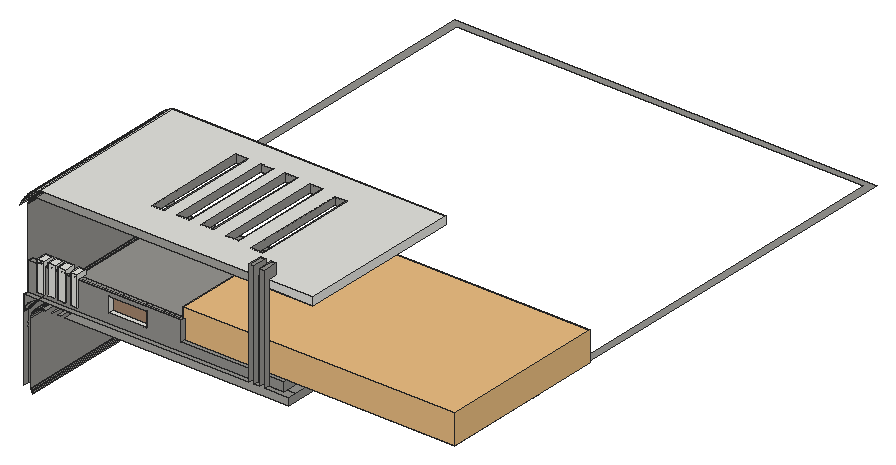
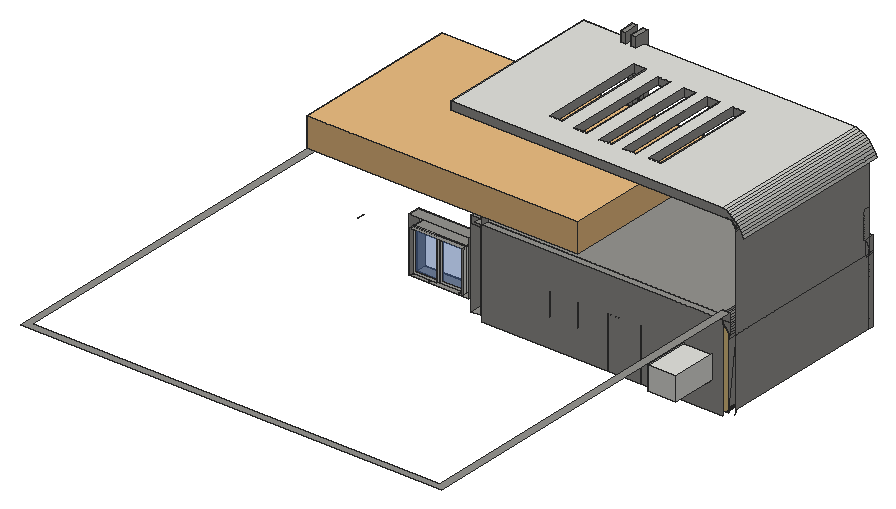
# SketchUp Ruby script. Lengths in millimetres.
U = 1.mm
M = Sketchup.active_model
def pt(a) = Geom::Point3d.new(a.map { |v| v * U })
def face(e, loops, mat)
  f = e.add_face(loops[0].map { |a| pt(a) })
  loops[1..].each { |l| e.add_face(l.map { |a| pt(a) }).erase! }
  f.material = f.back_material = mat if mat
  f
end
# faces: each face lists its corners as indices into pts; further lists are holes
def faces(e, pts, list, mat = nil) = list.each { |f| face(e, (f[0].is_a?(Array) ? f : [f]).map { |l| l.map { |i| pts[i] } }, mat) }
# xy, xz, yz: faces in a plane at the given z, y or x. An outline is a flat list of corners, or four numbers for a rectangle; further outlines are holes
def ring(l) = l.size == 4 ? [[l[0], l[1]], [l[2], l[1]], [l[2], l[3]], [l[0], l[3]]] : l.each_slice(2).to_a
def flat(e, list, mat, &to3) = list.each { |f| face(e, (f[0].is_a?(Array) ? f : [f]).map { |l| ring(l).map { |u, v| to3.(u, v) } }, mat) }
def xy(e, z, list, mat = nil) = flat(e, list, mat) { |x, y| [x, y, z] }
def xz(e, y, list, mat = nil) = flat(e, list, mat) { |x, z| [x, y, z] }
def yz(e, x, list, mat = nil) = flat(e, list, mat) { |y, z| [x, y, z] }
def lines(e, pts, list) = list.each { |a, b| e.add_line(pt(pts[a]), pt(pts[b])) }
# prism: a flat outline (further loops are holes) pulled along v
def prism(e, loops, v, mat = nil)
  f = face(e, loops, mat); d = Geom::Vector3d.new(v.map { |x| x * U })
  f.pushpull(f.normal.samedirection?(d) ? d.length : -d.length)
end
def box(e, o, s, mat = nil) = prism(e, [[o, [o[0] + s[0], o[1], o[2]], [o[0] + s[0], o[1] + s[1], o[2]], [o[0], o[1] + s[1], o[2]]]], [0, 0, s[2]], mat)
def at(x, y, z, deg = 0) = Geom::Transformation.translation(pt([x, y, z])) * Geom::Transformation.rotation(ORIGIN, Z_AXIS, deg.degrees)
def axes(o, x, y, z) = Geom::Transformation.new([*x, 0, *y, 0, *z, 0, *pt(o).to_a, 1])
def part(name) = M.definitions.add(name)
# library, detail: a bought-in or finely detailed component or shape, given as its bounding box
def library(name, o, s) = part(name).tap { |d| box(d.entities, o, s) }
def detail(e, o, s) = box(e.add_group.entities, o, s)
def put(e, d, t, mat = nil) = e.add_instance(d, t).tap { |i| i.material = mat if mat }
def group(e, t, mat = nil) = e.add_group.tap { |g| g.transformation = t; g.material = mat if mat }.entities
root = M.entities
M.materials.add("Polis06_194").color = [79, 50, 36]
M.materials.add("Teddy_BraceletShadow ").color = [165, 134, 109]
M.materials.add("[Granite Light Gray]").color = [149, 148, 144]
M.materials.add("[Stone Brushed Khaki]").color = [226, 197, 133]
M.materials.add("[Translucent Glass Blue]").color = [100, 149, 237]
M.materials["[Translucent Glass Blue]"].alpha = 0.5
c1 = part("Flush door")
xy(c1.entities,0,[[0,0,120,30],[0,870,120,900]],"Polis06_194")
xy(c1.entities,2165.6,[[0,30,120,870]],"Polis06_194")
xy(c1.entities,2200,[[0,0,120,900]],"Polis06_194")
xz(c1.entities,0,[[0,0,120,2200]],"Polis06_194")
xz(c1.entities,30,[[0,0,60,2165.6],[60,0,120,2165.6]],"Polis06_194")
xz(c1.entities,870,[[0,0,120,2165.6]],"Polis06_194")
xz(c1.entities,900,[[0,0,120,2200]],"Polis06_194")
yz(c1.entities,0,[[0,0,30,2200],[870,0,900,2200],[30,2165.6,870,2200]],"Polis06_194")
yz(c1.entities,60,[[30,0,870,0,870,2164.4,30,2165.6]],"Polis06_194")
yz(c1.entities,120,[[0,0,30,2200],[870,0,900,2200],[30,2165.6,870,2200]],"Polis06_194")
c2 = part("Janela aluminio")
xy(c2.entities,0,[[0,0,1200,40],[600,40,1200,70],[0,70,660,100],[0,100,1200,150]])
xy(c2.entities,1100,[[0,0,1200,40],[600,40,1200,70],[0,70,0,150,1200,150,1200,100,660,100,660,70],[660,70,1200,100]])
xz(c2.entities,40,[[0,0,600,0,600,1050,540,1050,540,50,50,50,50,1050,600,1050,600,1100,0,1100],[[600,0,1200,1100],[652.8,50,1150,1050]]])
xz(c2.entities,70,[[[0,0,600,1100],[60,60,540,1040]],[600,0,660,1100]])
xz(c2.entities,70,[[60,60,540,1040]],"[Translucent Glass Blue]")
xz(c2.entities,100,[[660,0,660,60,1140,60,1140,1040,660,1040,660,1100,1200,1100,1200,0]])
xz(c2.entities,100,[[660,60,1140,1040]],"[Translucent Glass Blue]")
yz(c2.entities,0,[[0,0,40,1100],[70,0,150,1100]])
yz(c2.entities,600,[[40,0,70,1100]])
yz(c2.entities,660,[[70,0,100,1100]])
yz(c2.entities,1200,[[0,0,40,1100],[40,0,70,1100],[100,0,150,1100]])
c3 = library("Group\#4",[0,0,0],[8860.2,5530.7,939.4])
prism(root,[[[6157.2,6014.3,4191],[5238.9,6013,4191],[5238.6,6241.6,4191],[6156.9,6242.9,4191]]],[0,0,762])
prism(root,[[[1778.8,7701.8,4191],[859.6,7700.5,4191],[861.7,6241.6,4191],[1780.9,6242.9,4191]]],[0,0,762])
xy(root,3629.7,[[8973.7,5611.8,10939,6015]],"[Granite Light Gray]")
xy(root,3805.2,[[9005,5611.8,10719.5,6243.6]],"[Granite Light Gray]")
xy(root,5181.6,[[9005,5611.8,10719.5,6243.6]],"[Granite Light Gray]")
xy(root,5406.1,[[8973.7,5611.8,10939,6015]],"[Granite Light Gray]")
xy(root,5840.1,[[716.7,442.9,905.1,731.8]],"[Granite Light Gray]")
xy(root,5867.4,[[856.5,442.9,856.5,6013,8897.2,6013,8897.2,442.9,1577.5,442.9,1577.5,731.8,1445.7,731.8,1445.7,442.9,1348.7,442.9,1348.7,731.8,1205.9,731.8,1205.9,442.9,1150.1,442.9,1150.1,731.8,961.7,731.8,961.7,442.9],[8592.4,6013,8897.2,6013.2]],"[Granite Light Gray]")
xy(root,6037.3,[[718.4,792.9,8517,6013]],"[Granite Light Gray]")
xy(root,6096,[[254,435,718.4,435,718.4,442.9,7588,442.9,7588,604.8,254,604.8],[7749.9,442.9,7934.7,604.8],[8096.7,442.9,8897.2,442.9,8897.2,731.8,8592.4,731.8,8592.4,604.8,8096.7,604.8],[254,604.8,718.4,731.8],[718.4,604.8,8592.4,604.8,8592.4,6013,8517,6013,8517,792.9,718.4,792.9],
  [254,731.8,718.4,792.9],[8592.4,731.8,8897.2,6013],[718.4,792.9,8517,6013],[482.6,6013,8592.4,6013,8592.4,6015,8363.8,6015,8363.8,6243.6,482.6,6243.6],[8363.8,6015,8592.4,6243.6]],"[Granite Light Gray]")
xy(root,6202.4,[[569.6,579.4,793.4,604.8],[1239.8,579.4,1498,604.8],[1659.7,579.4,1880,604.8]],"[Granite Light Gray]")
xy(root,6378.2,[[5236.2,604.8,8592.4,604.8,8592.4,6013,8517,6013,8517,792.9,5236.2,792.9],[8363.8,6015,13995.4,6015,13995.4,18029.2,254,18029.2,254,6243.6,482.6,6243.6,482.6,17800.6,13766.8,17800.6,13766.8,6243.6,8363.8,6243.6]],"[Granite Light Gray]")
xy(root,6400.8,[[2891.4,604.8,4124.9,776.3]])
xy(root,6891.3,[[2891.4,604.8,4124.9,776.3]])
xy(root,7010.4,[[254,604.8,569.6,604.8,569.6,731.8,565.7,792.9,254,792.9],[793.4,604.8,902.8,792.9],[1150.4,604.8,1239.8,792.9],[1498,604.8,1659.7,792.9],[1880,604.8,5236.2,792.9],
  [565.7,792.9,793.4,929.5],[902.8,792.9,910.7,929.5],[910.7,792.9,1150.4,929.5],[1239.8,792.9,1498,929.5],[1659.7,792.9,1880,929.5]],"[Granite Light Gray]")
xy(root,7162.8,[[569.6,579.4,793.4,579.4,793.4,929.5,565.7,929.5,565.7,792.9,569.6,731.8],[1239.8,579.4,1498,929.5],[1659.7,579.4,1880,929.5],[902.8,604.8,1150.4,929.5]])
xy(root,8946.3,[[[544.6,604.8,9558.3,6015],[4960,1775.3,5361.6,5205.9],[4181.7,1772.3,4583.3,5202.9],[6705.3,1605.8,7106.9,5036.4],[5823.4,1719.2,6225,5149.8],[3362.3,1753.6,3764,5184.2]]],"[Granite Light Gray]")
xy(root,9200.3,[[[665.2,604.8,7588,604.8,7588,917.6,7749.9,917.6,7749.9,604.8,7934.7,604.8,7934.7,917.6,8096.7,917.6,8096.7,604.8,9558.3,604.8,9558.3,6015,665.2,6015],[4960,1775.3,5361.6,5205.9],[4181.7,1772.3,4583.3,5202.9],[5823.4,1719.2,6225,5149.8],[6705.3,1605.8,7106.9,5036.4],[3362.3,1753.6,3764,5184.2]]])
xy(root,9200.3,[[7588,604.8,7749.9,917.6],[7934.7,604.8,8096.7,917.6]],"[Granite Light Gray]")
xy(root,9540.9,[[7588,442.9,7749.9,917.6],[7934.7,442.9,8096.7,917.6]],"[Granite Light Gray]")
xz(root,435,[[254,5579.2,289.9,5624.7,326.4,5669.7,363.3,5714.3,400.8,5758.5,438.8,5802.3,477.3,5845.6,516.3,5888.5,555.7,5930.9,595.7,5972.9,636.1,6014.4,677,6055.4,718.4,6096,665.5,6075.7,614.2,6051.5,565,6023.4,518,5991.7,473.6,5956.5,432,5918,393.5,5876.4,358.3,5832,326.6,5785,298.5,5735.8,274.3,5684.5,254,5631.6],[254,5631.6,274.3,5684.5,298.5,5735.8,326.6,5785,358.3,5832,393.5,5876.4,432,5918,473.6,5956.5,518,5991.7,565,6023.4,614.2,6051.5,665.5,6075.7,718.4,6096,254,6096]],"[Granite Light Gray]")
xz(root,579.4,[[569.6,6202.4,793.4,7162.8],[1239.8,6202.4,1498,7162.8],[1659.7,6202.4,1880,7162.8]])
xz(root,604.8,[[902.8,6202.4,1150.4,7162.8],[7749.9,8946.3,7934.7,9200.3],[8096.7,8946.3,9558.3,9200.3]])
xz(root,604.8,[[[254,6096,7588,6096,7588,6378.2,5236.2,6378.2,5236.2,7010.4,1880,7010.4,1880,6202.4,1659.7,6202.4,1659.7,7010.4,1498,7010.4,1498,6202.4,1239.8,6202.4,1239.8,7010.4,1150.4,7010.4,1150.4,6202.4,902.8,6202.4,902.8,7010.4,793.4,7010.4,793.4,6202.4,569.6,6202.4,569.6,7010.4,254,7010.4],[2891.4,6400.8,4124.9,6891.3]],[7588,6096,7749.9,6378.2],[7749.9,6096,7934.7,6378.2],[7934.7,6096,8096.7,6378.2],[8096.7,6096,8592.4,6378.2],
  [7588,6378.2,7749.9,8946.3],[7934.7,6378.2,8096.7,8946.3],[7588,8946.3,7749.9,9200.3],[7934.7,8946.3,8096.7,9200.3]],"[Granite Light Gray]")
xz(root,731.8,[[254,5579.2,254,6096,718.4,6096,677,6055.4,636.1,6014.4,595.7,5972.9,555.7,5930.9,516.3,5888.5,477.3,5845.6,438.8,5802.3,400.8,5758.5,363.3,5714.3,326.4,5669.7,289.9,5624.7]],"[Granite Light Gray]")
xz(root,776.3,[[2891.4,6400.8,4124.9,6891.3]],"Teddy_BraceletShadow ")
xz(root,792.9,[[718.4,6037.3,8517,6096],[254,6096,254,7010.4,5236.2,7010.4,5236.2,6378.2,8517,6378.2,8517,6096]],"[Granite Light Gray]")
xz(root,917.6,[[7588,9200.3,7749.9,9540.9],[7934.7,9200.3,8096.7,9540.9]],"[Granite Light Gray]")
xz(root,929.5,[[565.7,7010.4,793.4,7162.8],[902.8,7010.4,1150.4,7162.8],[1239.8,7010.4,1498,7162.8],[1659.7,7010.4,1880,7162.8]],"[Granite Light Gray]")
xz(root,1605.8,[[6705.3,8946.3,7106.9,9200.3]],"[Granite Light Gray]")
xz(root,1719.2,[[5823.4,8946.3,6225,9200.3]],"[Granite Light Gray]")
xz(root,1753.6,[[3362.3,8946.3,3764,9200.3]],"[Granite Light Gray]")
xz(root,1772.3,[[4181.7,8946.3,4583.3,9200.3]],"[Granite Light Gray]")
xz(root,1775.3,[[4960,8946.3,5361.6,9200.3]],"[Granite Light Gray]")
xz(root,5036.4,[[6705.3,8946.3,7106.9,9200.3]],"[Granite Light Gray]")
xz(root,5149.8,[[5823.4,8946.3,6225,9200.3]],"[Granite Light Gray]")
xz(root,5184.2,[[3362.3,8946.3,3764,9200.3]],"[Granite Light Gray]")
xz(root,5202.9,[[4181.7,8946.3,4583.3,9200.3]],"[Granite Light Gray]")
xz(root,5205.9,[[4960,8946.3,5361.6,9200.3]],"[Granite Light Gray]")
xz(root,5611.8,[[[8973.7,3629.7,10939,5406.1],[9005,3805.2,10719.5,5181.6]]])
xz(root,6013,[[482.6,5493.5,482.6,5867.4,856.5,5867.4,807.7,5864.2,759.7,5854.7,713.4,5838.9,669.5,5817.3,628.9,5790.1,592.1,5757.9,559.9,5721.1,532.7,5680.5,511.1,5636.6,495.3,5590.3,485.8,5542.3],[482.6,5867.4,482.6,5963.6,518,5991.7,565,6023.4,614.2,6051.5,665.5,6075.7,718.4,6096,718.4,6037.3,8363.8,6037.3,8363.8,5867.4],[8363.8,5867.4,8363.8,6037.3,8517,6037.3,8517,6096,8897.2,6096,8897.2,5867.4],[482.6,5963.6,518,5991.7,565,6023.4,614.2,6051.5,665.5,6075.7,718.4,6096,482.6,6096],[718.4,6037.3,8363.8,6096],
  [8363.8,6037.3,8517,6096],[8517,6096,8592.4,6378.2]],"[Granite Light Gray]")
xz(root,6014.8,[[551.2,3269,482.6,3341.1,482.6,3423.3,484.6,3404,490.6,3373.9,500.4,3344.9,514,3317.5,531,3292],[484.6,3404,482.6,3423.3,482.6,3434.5],[484.6,3404,482.6,3423.3,482.6,3434.5],[484.6,3404,482.6,3423.3,482.6,3434.5]],"[Granite Light Gray]")
xz(root,6015,[[254,8655.7,254,8946.3,544.6,8946.3,506.7,8943.8,469.4,8936.4,433.4,8924.2,399.3,8907.4,367.7,8886.3,339.1,8861.2,314.1,8832.6,292.9,8801,276.1,8766.9,263.9,8730.9,256.5,8693.6],[254,8946.3,313.6,9001.5,377.4,9051.9,444.8,9097.3,515.6,9137.3,589.2,9171.7,665.2,9200.3,9558.3,9200.3,9558.3,8946.3]],"[Granite Light Gray]")
xz(root,6243.6,[[482.6,3276.6,8363.8,6096],[254,5631.6,274.3,5684.5,298.5,5735.8,326.6,5785,358.3,5832,393.5,5876.4,432,5918,473.6,5956.5,482.6,5963.6,482.6,6096,254,6096],[254,6096,482.6,6378.2]],"[Granite Light Gray]")
yz(root,254,[[442.9,3432.9,604.8,5579.2],[604.8,3432.9,6015,3432.9,6015,5631.6,731.8,5631.6,731.8,5579.2,604.8,5579.2],[435,5579.2,604.8,5631.6],[604.8,5579.2,731.8,5631.6],[435,5631.6,435,6096,604.8,6096,604.8,5820.7,517.6,5631.6],
  [517.6,5631.6,604.8,5820.7,604.8,5631.6],[604.8,5631.6,731.8,5631.6,731.8,6096,604.8,5820.7],[731.8,5631.6,6015,5631.6,6015,8655.7,604.8,8655.7,604.8,7010.4,792.9,7010.4,792.9,6096,731.8,6096],[604.8,5820.7,604.8,6096,731.8,6096],[604.8,6096,792.9,7010.4]],"[Granite Light Gray]")
yz(root,482.6,[[6014.8,3276.6,6014.9,3276.6,6014.8,3423.3],[442.9,3434.5,6014.8,3434.5,6013.1,5963.6,6013,5963.6,6013,5493.5,442.9,5493.5],[6013,5963.6,6013.1,5963.6,6013,6096],[6013.1,5963.6,6013,6096,6243.6,6096,6243.6,5963.6],[759.9,6954.2,764.5,6954.8,768.7,6956.6,772.3,6959.3,775.1,6962.9,776.8,6967.2,777.4,6971.7,776.8,6976.2,775.1,6980.4,772.3,6984,768.7,6986.8,764.5,6988.5,759.9,6989.1,755.4,6988.5,751.2,6986.8,747.6,6984,744.8,6980.4,743.1,6976.2,742.5,6971.7,743.1,6967.2,744.8,6962.9,747.6,6959.3,751.2,6956.6,755.4,6954.8]],"[Granite Light Gray]")
yz(root,565.7,[[792.9,7010.4,929.5,7162.8]])
yz(root,569.6,[[579.4,6202.4,579.4,7162.8,731.8,7162.8,731.8,7010.4,604.8,7010.4,604.8,6202.4]])
yz(root,718.4,[[792.9,6037.3,6013,6096]],"[Granite Light Gray]")
yz(root,793.4,[[579.4,6202.4,604.8,6202.4,604.8,7010.4,929.5,7010.4,929.5,7162.8,579.4,7162.8]])
yz(root,902.8,[[604.8,7010.4,731.8,7162.8],[731.8,7010.4,929.5,7162.8]])
yz(root,1150.4,[[604.8,7010.4,929.5,7162.8]])
yz(root,1239.8,[[579.4,6202.4,579.4,7162.8,731.8,7162.8,731.8,7010.4,604.8,7010.4,604.8,6202.4],[731.8,7010.4,929.5,7162.8]])
yz(root,1498,[[579.4,6202.4,604.8,6202.4,604.8,7010.4,929.5,7010.4,929.5,7162.8,579.4,7162.8]])
yz(root,1659.7,[[579.4,6202.4,579.4,7162.8,731.8,7162.8,731.8,7010.4,604.8,7010.4,604.8,6202.4],[731.8,7010.4,929.5,7162.8]])
yz(root,1880,[[579.4,6202.4,604.8,6202.4,604.8,7010.4,929.5,7010.4,929.5,7162.8,579.4,7162.8]])
yz(root,2891.4,[[604.8,6400.8,776.3,6891.3]])
yz(root,3170.2,[[6014.9,3276.6,6243.5,3276.8,6242.4,4963.4,6013.8,4963.2]],"[Granite Light Gray]")
yz(root,3362.3,[[1753.6,8946.3,5184.2,9200.3]],"[Granite Light Gray]")
yz(root,3764,[[1753.6,8946.3,5184.2,9200.3]],"[Granite Light Gray]")
yz(root,4124.9,[[604.8,6400.8,776.3,6891.3]])
yz(root,4181.7,[[1772.3,8946.3,5202.9,9200.3]],"[Granite Light Gray]")
yz(root,4237,[[6014.9,3276.6,6013.8,4963.2,6242.4,4963.4,6243.5,3276.8]],"[Granite Light Gray]")
yz(root,4583.3,[[1772.3,8946.3,5202.9,9200.3]],"[Granite Light Gray]")
yz(root,4960,[[1775.3,8946.3,5205.9,9200.3]],"[Granite Light Gray]")
yz(root,5236.2,[[[604.8,6378.2,792.9,7010.4],[759.9,6954.2,755.4,6954.8,751.2,6956.6,747.6,6959.3,744.8,6962.9,743.1,6967.2,742.5,6971.7,743.1,6976.2,744.8,6980.4,747.6,6984,751.2,6986.8,755.4,6988.5,759.9,6989.1,764.5,6988.5,768.7,6986.8,772.3,6984,775.1,6980.4,776.8,6976.2,777.4,6971.7,776.8,6967.2,775.1,6962.9,772.3,6959.3,768.7,6956.6,764.5,6954.8]],[759.9,6954.2,764.5,6954.8,768.7,6956.6,772.3,6959.3,775.1,6962.9,776.8,6967.2,777.4,6971.7,776.8,6976.2,775.1,6980.4,772.3,6984,768.7,6986.8,764.5,6988.5,759.9,6989.1,755.4,6988.5,751.2,6986.8,747.6,6984,744.8,6980.4,743.1,6976.2,742.5,6971.7,743.1,6967.2,744.8,6962.9,747.6,6959.3,751.2,6956.6,755.4,6954.8]],"[Granite Light Gray]")
yz(root,5361.6,[[1775.3,8946.3,5205.9,9200.3]],"[Granite Light Gray]")
yz(root,5823.4,[[1719.2,8946.3,5149.8,9200.3]],"[Granite Light Gray]")
yz(root,6225,[[1719.2,8946.3,5149.8,9200.3]],"[Granite Light Gray]")
yz(root,6705.3,[[1605.8,8946.3,5036.4,9200.3]],"[Granite Light Gray]")
yz(root,7106.9,[[1605.8,8946.3,5036.4,9200.3]],"[Granite Light Gray]")
yz(root,7588,[[442.9,6096,442.9,9540.9,917.6,9540.9,917.6,9200.3,604.8,9200.3,604.8,6096]],"[Granite Light Gray]")
yz(root,7749.9,[[442.9,6096,604.8,6096,604.8,9200.3,917.6,9200.3,917.6,9540.9,442.9,9540.9]],"[Granite Light Gray]")
yz(root,7934.7,[[442.9,6096,442.9,9540.9,917.6,9540.9,917.6,9200.3,604.8,9200.3,604.8,6096]],"[Granite Light Gray]")
yz(root,8096.7,[[442.9,6096,604.8,6096,604.8,9200.3,917.6,9200.3,917.6,9540.9,442.9,9540.9]],"[Granite Light Gray]")
yz(root,8363.8,[[6015,6096,6243.6,6378.2]],"[Granite Light Gray]")
yz(root,8517,[[792.9,6037.3,6013,6096],[792.9,6096,6013,6378.2]],"[Granite Light Gray]")
yz(root,8592.4,[[5557.7,3276.3,6014.9,3276.6,6013.2,5867.4,6013,5867.4,5556,5867.1],[604.8,6096,6013,6378.2]],"[Granite Light Gray]")
yz(root,8897.2,[[5557.7,3276.3,5556,5867.1,6013,5867.4,6013.2,5867.4,6014.9,3276.6],[442.9,5867.4,6013,6096]],"[Granite Light Gray]")
yz(root,8973.7,[[5611.8,3629.7,6015,5406.1]],"[Granite Light Gray]")
yz(root,9005,[[5611.8,3805.2,6243.6,5181.6]],"[Granite Light Gray]")
yz(root,9558.3,[[604.8,8946.3,6015,9200.3]])
yz(root,10719.5,[[5611.8,3805.2,6243.6,5181.6]],"[Granite Light Gray]")
yz(root,10939,[[5611.8,3629.7,6015,5406.1]],"[Granite Light Gray]")
yz(root,12406.8,[[6015,4875.3,6243.6,4876.8]])
p = [[531,6014.8,3292],[531,442.9,3292],[551.2,442.9,3269],[551.2,6014.8,3269],[8897.2,5557.7,3276.3],[8592.4,5557.7,3276.3],
  [8592.4,5556,5867.1],[8897.2,5556,5867.1],[8897.2,6014.9,3276.6],[8592.4,6014.9,3276.6],[482.6,6014.9,3276.6],[3170.2,6014.9,3276.6],
  [3170.2,6013.8,4963.2],[4237,6013.8,4963.2],[4237,6014.9,3276.6],[8592.4,6013.2,5867.4],[8592.4,6013,6096],[8517,6013,6096],
  [8363.8,6013,6096],[718.4,6013,6096],[482.6,6013,6096],[482.6,6013.1,5963.6],[482.6,6014.8,3434.5],[482.6,6014.8,3423.3],
  [4237,6243.5,3276.8],[3170.2,6243.5,3276.8],[4237,6242.4,4963.4],[3170.2,6242.4,4963.4],[294.3,6015,3288.9],[294.3,6014.8,3288.9],
  [269.9,6014.8,3359.7],[269.9,6015,3359.7],[514,6014.8,3317.5],[514,442.9,3317.5],[500.4,6014.8,3344.9],[500.4,442.9,3344.9],
  [490.6,6014.8,3373.9],[490.6,442.9,3373.9],[254,6014.8,3432.9],[254,6015,3432.9],[484.6,6014.8,3404],[484.6,442.9,3404],
  [482.6,442.9,3434.5],[485.8,6013,5542.3],[485.8,442.9,5542.3],[482.6,442.9,5493.5],[482.6,6013,5493.5],[495.3,6013,5590.3],
  [495.3,442.9,5590.3],[289.9,435,5624.7],[254,435,5579.2],[254,442.9,5579.2],[289.9,442.9,5624.7],[254,731.8,5579.2],
  [289.9,731.8,5624.7],[254,604.8,5579.2],[511.1,6013,5636.6],[511.1,442.9,5636.6],[326.4,435,5669.7],[326.4,442.9,5669.7],
  [326.4,731.8,5669.7],[254,6015,5631.6],[254,731.8,5631.6],[254,604.8,5631.6],[254,517.6,5631.6],[254,435,5631.6],
  [274.3,435,5684.5],[274.3,6243.6,5684.5],[254,6243.6,5631.6],[532.7,6013,5680.5],[532.7,442.9,5680.5],[363.3,435,5714.3],
  [363.3,442.9,5714.3],[363.3,731.8,5714.3],[559.9,6013,5721.1],[559.9,442.9,5721.1],[298.5,435,5735.8],[298.5,6243.6,5735.8],
  [400.8,435,5758.5],[400.8,442.9,5758.5],[400.8,731.8,5758.5],[592.1,6013,5757.9],[592.1,442.9,5757.9],[326.6,435,5785],
  [326.6,6243.6,5785],[628.9,6013,5790.1],[628.9,442.9,5790.1],[438.8,435,5802.3],[438.8,442.9,5802.3],[438.8,731.8,5802.3],
  [358.3,435,5832],[358.3,6243.6,5832],[669.5,6013,5817.3],[669.5,442.9,5817.3],[477.3,435,5845.6],[477.3,442.9,5845.6],
  [477.3,731.8,5845.6],[713.4,6013,5838.9],[713.4,442.9,5838.9],[393.5,435,5876.4],[393.5,6243.6,5876.4],[759.7,6013,5854.7],
  [759.7,442.9,5854.7],[716.7,442.9,5840.1],[516.3,435,5888.5],[516.3,442.9,5888.5],[516.3,731.8,5888.5],[807.7,6013,5864.2],
  [807.7,442.9,5864.2],[856.5,6013,5867.4],[856.5,442.9,5867.4],[8592.4,6013,5867.4],[8897.2,6013,5867.4],[432,435,5918],
  [432,6243.6,5918],[555.7,435,5930.9],[555.7,442.9,5930.9],[555.7,731.8,5930.9],[473.6,435,5956.5],[473.6,6243.6,5956.5],
  [595.7,435,5972.9],[595.7,442.9,5972.9],[595.7,731.8,5972.9],[518,435,5991.7],[518,6013,5991.7],[482.6,6013,5963.6],
  [482.6,6243.6,5963.6],[636.1,435,6014.4],[636.1,442.9,6014.4],[636.1,731.8,6014.4],[565,435,6023.4],[565,6013,6023.4],
  [677,435,6055.4],[677,442.9,6055.4],[677,731.8,6055.4],[614.2,435,6051.5],[614.2,6013,6051.5],[665.5,435,6075.7],
  [665.5,6013,6075.7],[718.4,435,6096],[718.4,442.9,6096],[5236.2,755.4,6954.8],[5236.2,759.9,6954.2],[482.6,759.9,6954.2],
  [482.6,755.4,6954.8],[5236.2,764.5,6954.8],[482.6,764.5,6954.8],[5236.2,751.2,6956.6],[482.6,751.2,6956.6],[5236.2,768.7,6956.6],
  [482.6,768.7,6956.6],[5236.2,747.6,6959.3],[482.6,747.6,6959.3],[5236.2,772.3,6959.3],[482.6,772.3,6959.3],[5236.2,744.8,6962.9],
  [482.6,744.8,6962.9],[5236.2,775.1,6962.9],[482.6,775.1,6962.9],[5236.2,743.1,6967.2],[482.6,743.1,6967.2],[5236.2,776.8,6967.2],
  [482.6,776.8,6967.2],[5236.2,742.5,6971.7],[482.6,742.5,6971.7],[5236.2,777.4,6971.7],[482.6,777.4,6971.7],[5236.2,743.1,6976.2],
  [482.6,743.1,6976.2],[5236.2,776.8,6976.2],[482.6,776.8,6976.2],[5236.2,744.8,6980.4],[482.6,744.8,6980.4],[5236.2,775.1,6980.4],
  [482.6,775.1,6980.4],[5236.2,747.6,6984],[482.6,747.6,6984],[5236.2,772.3,6984],[482.6,772.3,6984],[5236.2,751.2,6986.8],
  [482.6,751.2,6986.8],[5236.2,768.7,6986.8],[482.6,768.7,6986.8],[5236.2,755.4,6988.5],[482.6,755.4,6988.5],[5236.2,764.5,6988.5],
  [482.6,764.5,6988.5],[5236.2,759.9,6989.1],[482.6,759.9,6989.1],[565.7,792.9,7010.4],[569.6,731.8,7010.4],[569.6,731.8,7162.8],
  [565.7,792.9,7162.8],[0,6015,8535.1],[0,604.8,8535.1],[28.6,604.8,8611.1],[28.6,6015,8611.1],[63,604.8,8684.8],
  [63,6015,8684.8],[256.5,6015,8693.6],[256.5,604.8,8693.6],[254,604.8,8655.7],[254,6015,8655.7],[103,604.8,8755.5],
  [103,6015,8755.5],[263.9,6015,8730.9],[263.9,604.8,8730.9],[276.1,6015,8766.9],[276.1,604.8,8766.9],[148.4,604.8,8822.9],
  [148.4,6015,8822.9],[292.9,6015,8801],[292.9,604.8,8801],[314.1,6015,8832.6],[314.1,604.8,8832.6],[198.8,604.8,8886.7],
  [198.8,6015,8886.7],[339.1,6015,8861.2],[339.1,604.8,8861.2],[367.7,6015,8886.3],[367.7,604.8,8886.3],[399.3,6015,8907.4],
  [399.3,604.8,8907.4],[254,604.8,8946.3],[254,6015,8946.3],[433.4,6015,8924.2],[433.4,604.8,8924.2],[469.4,6015,8936.4],
  [469.4,604.8,8936.4],[506.7,6015,8943.8],[506.7,604.8,8943.8],[544.6,6015,8946.3],[544.6,604.8,8946.3],[313.6,604.8,9001.5],
  [313.6,6015,9001.5],[377.4,604.8,9051.9],[377.4,6015,9051.9],[444.8,604.8,9097.3],[444.8,6015,9097.3],[515.6,604.8,9137.3],
  [515.6,6015,9137.3],[589.2,604.8,9171.7],[589.2,6015,9171.7],[665.2,604.8,9200.3],[665.2,6015,9200.3],[482.6,6013,5867.4],
  [482.6,731.8,5867.4],[8592.4,6013,7010.4],[8592.4,6015,7010.4]]
faces(root,p,[[0,1,2,3],[4,5,6,7],[8,9,5,4],[11,14,24,25],[25,24,26,27],[28,29,30,31],[32,33,1,0],[34,35,33,32],
  [36,37,35,34],[31,30,38,39],[40,41,37,36],[22,42,41,40],[13,12,27,26],[43,44,45,46],[47,48,44,43],[49,50,51,52],
  [53,54,52,51,55],[56,57,48,47],[58,49,52,59],[54,60,59,52],[61,62,63,64,65,66,67,68],[69,70,57,56],[71,58,59,72],[60,73,72,59],
  [74,75,70,69],[67,66,76,77],[78,71,72,79],[73,80,79,72],[81,82,75,74],[77,76,83,84],[85,86,82,81],[87,78,79,88],
  [80,89,88,79],[84,83,90,91],[92,93,86,85],[94,87,88,95],[89,96,95,88],[97,98,93,92],[91,90,99,100],[101,102,103,98,97],
  [104,94,95,105],[96,106,105,95],[107,108,102,101],[109,110,108,107],[6,111,112,7],[100,99,113,114],[115,104,105,116],[106,117,116,105],
  [114,113,118,119],[120,115,116,121],[117,122,121,116],[119,118,123,124,125,21,126],[127,120,121,128],[122,129,128,121],[124,123,130,131],[132,127,128,133],
  [129,134,133,128],[131,130,135,136],[136,135,137,138],[139,132,133,140],[141,142,143,144],[142,145,146,143],[147,141,144,148],[145,149,150,146],
  [151,147,148,152],[149,153,154,150],[155,151,152,156],[153,157,158,154],[159,155,156,160],[157,161,162,158],[163,159,160,164],[161,165,166,162],
  [167,163,164,168],[165,169,170,166],[171,167,168,172],[169,173,174,170],[175,171,172,176],[173,177,178,174],[179,175,176,180],[177,181,182,178],
  [183,179,180,184],[181,185,186,182],[187,183,184,188],[185,187,188,186],[199,200,201,202],[205,206,200,199],[207,208,206,205],[211,212,208,207],
  [213,214,212,211],[217,218,214,213],[219,220,218,217],[221,222,220,219],[225,226,222,221],[227,228,226,225],[229,230,228,227],[231,232,230,229]],"[Granite Light Gray]")
faces(root,p,[[10,11,12,13,14,9,15,16,17,18,19,20,21,22,23]],"[Stone Brushed Khaki]")
faces(root,p,[[189,190,191,192],[193,194,195,196],[196,195,197,198],[198,197,203,204],[204,203,209,210],[210,209,215,216],[216,215,223,224],[224,223,233,234],
  [234,233,235,236],[236,235,237,238],[238,237,239,240],[240,239,241,242],[242,241,243,244]])
lines(root,p,[[245,246],[23,61],[247,248]])
put(root,c1,axes([4237,6013.8,3276.6],[0,1.00935,0],[-1.18534,0,0],[0,0,0.76664]))
put(root,c2,axes([9005,6015,3805.2],[1.42875,0,0],[0,1,0],[0,0,1.25124]))
put(root,c2,axes([862,6489.6,4191],[0.75,0,0],[0,-2.17709,0],[0,0,0.59]))
put(root,c2,axes([5238.9,5887,4191],[1,0,0],[0,1.84,0],[0,0,0.68]))
put(root,c3,at(5186.2,752.9,6378.2))
